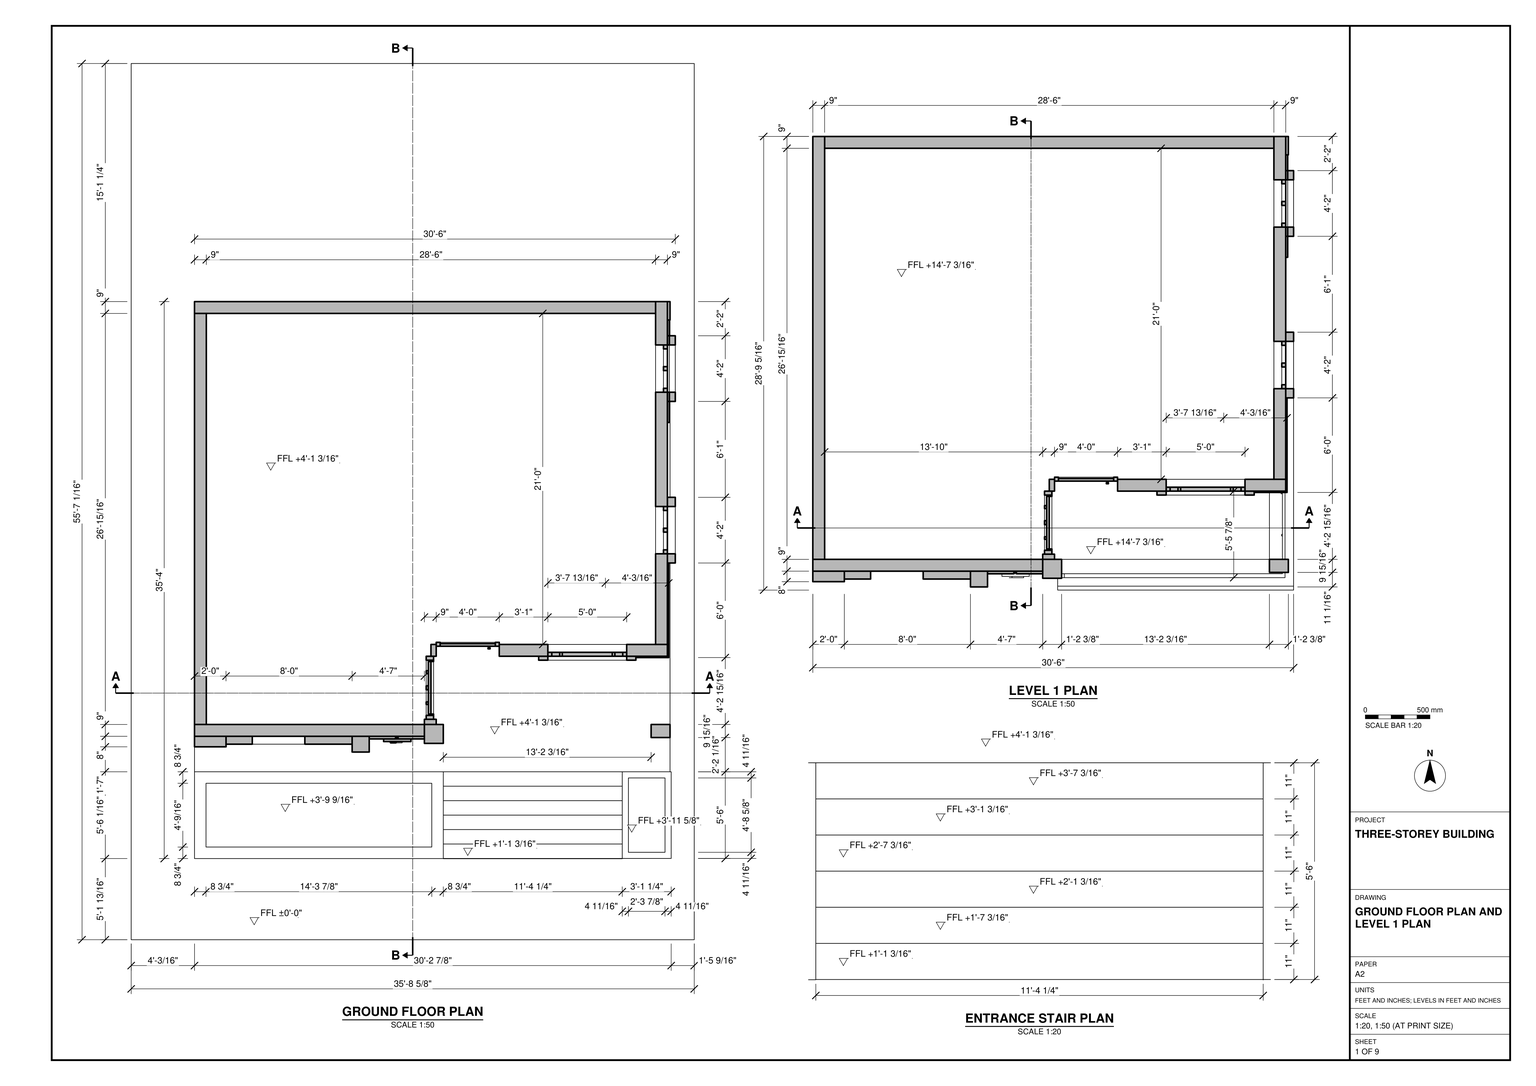
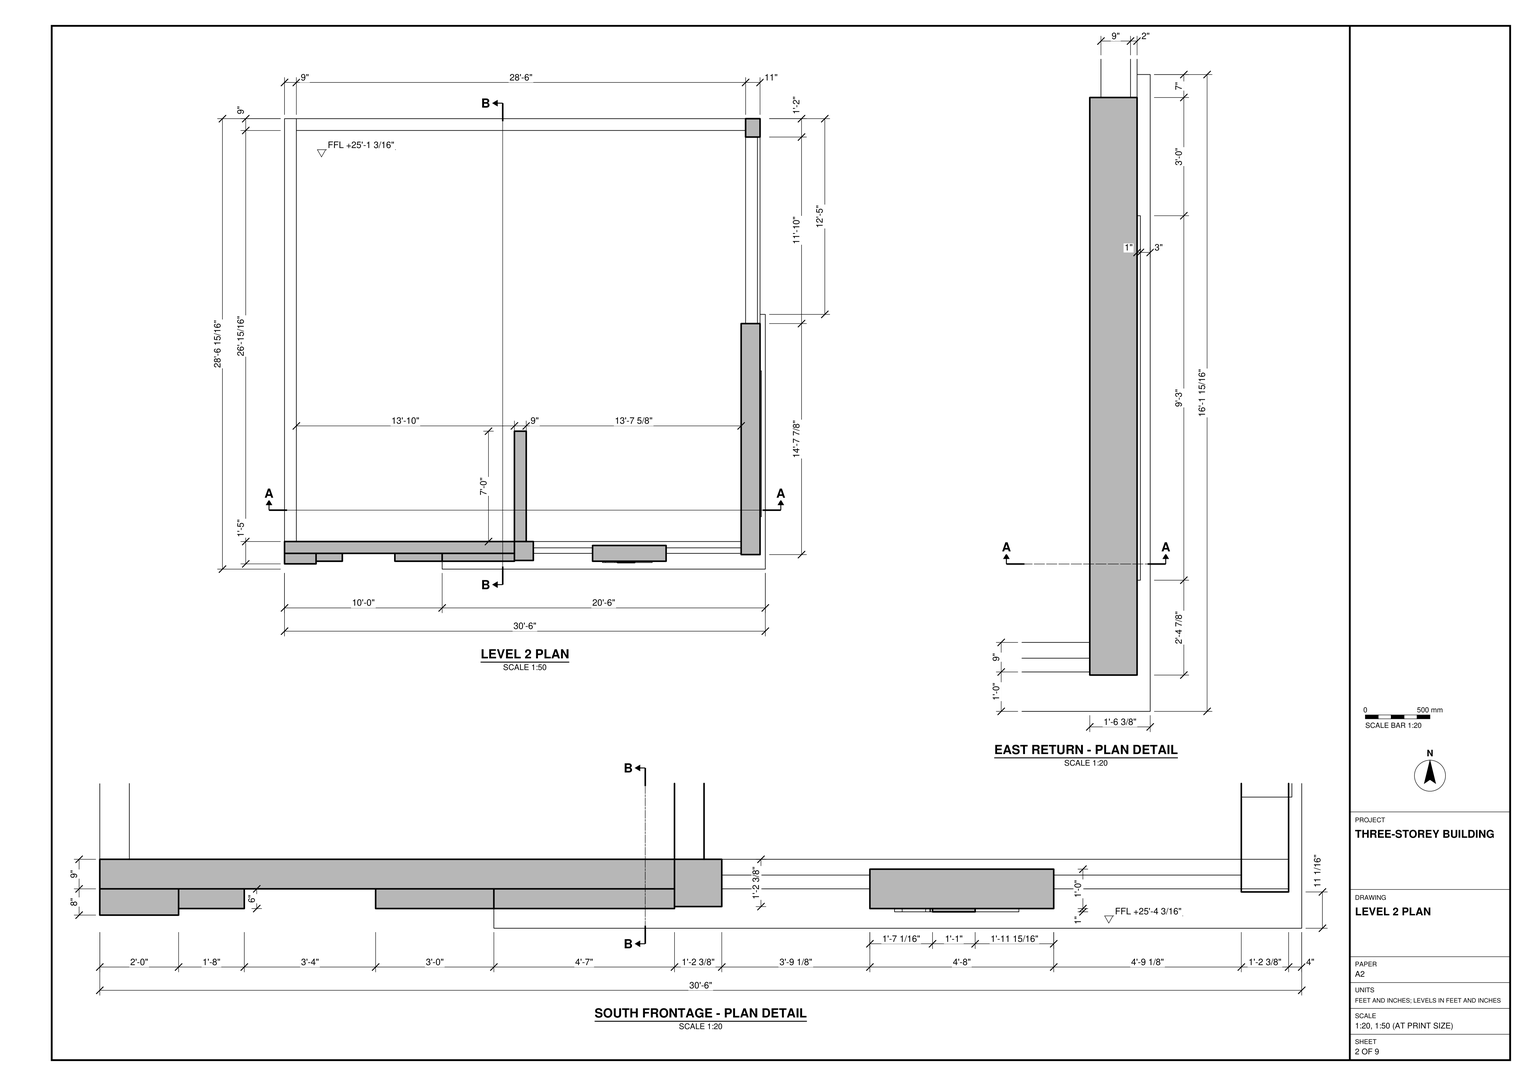
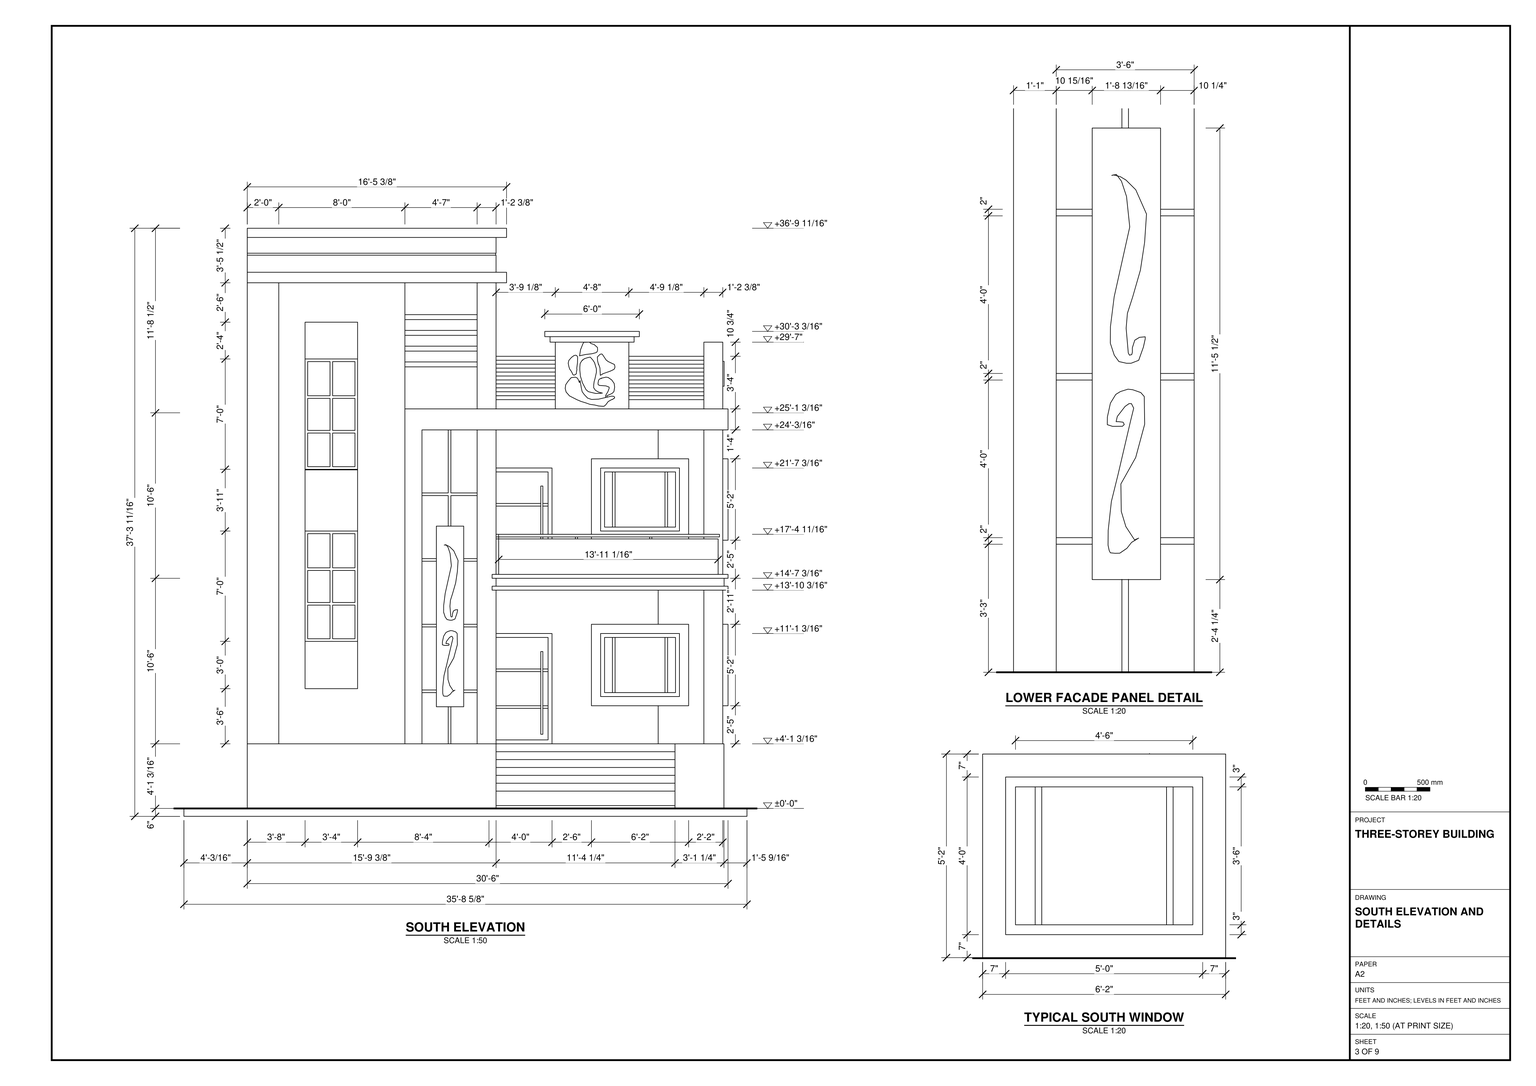
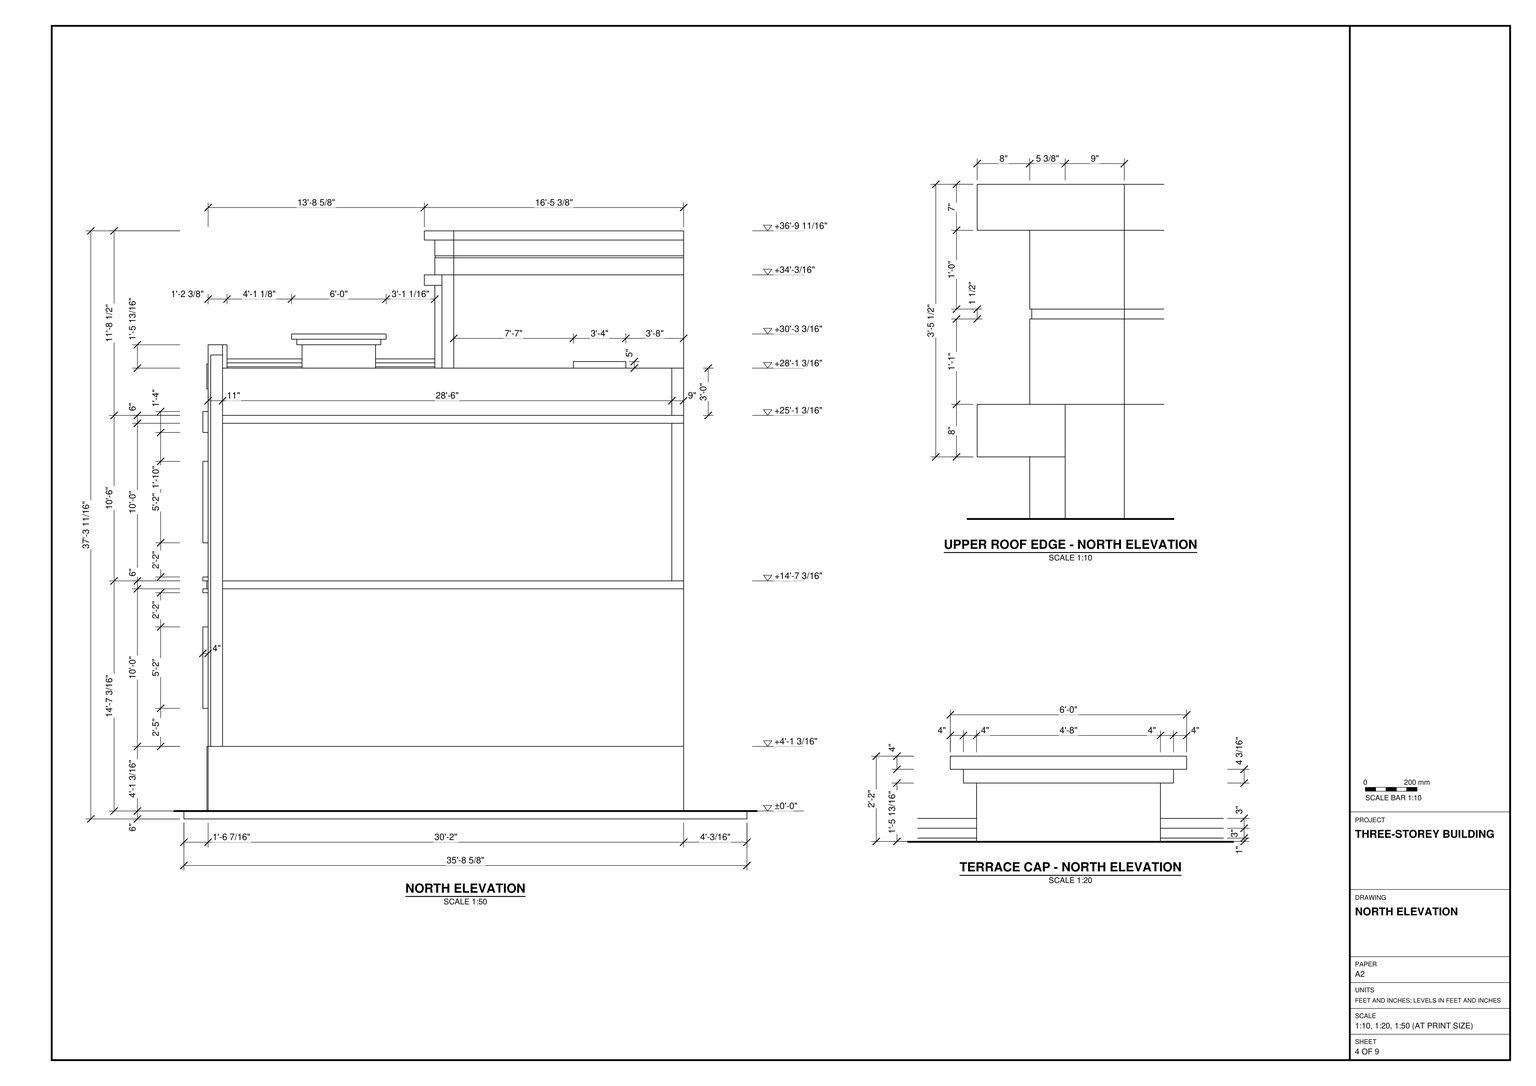
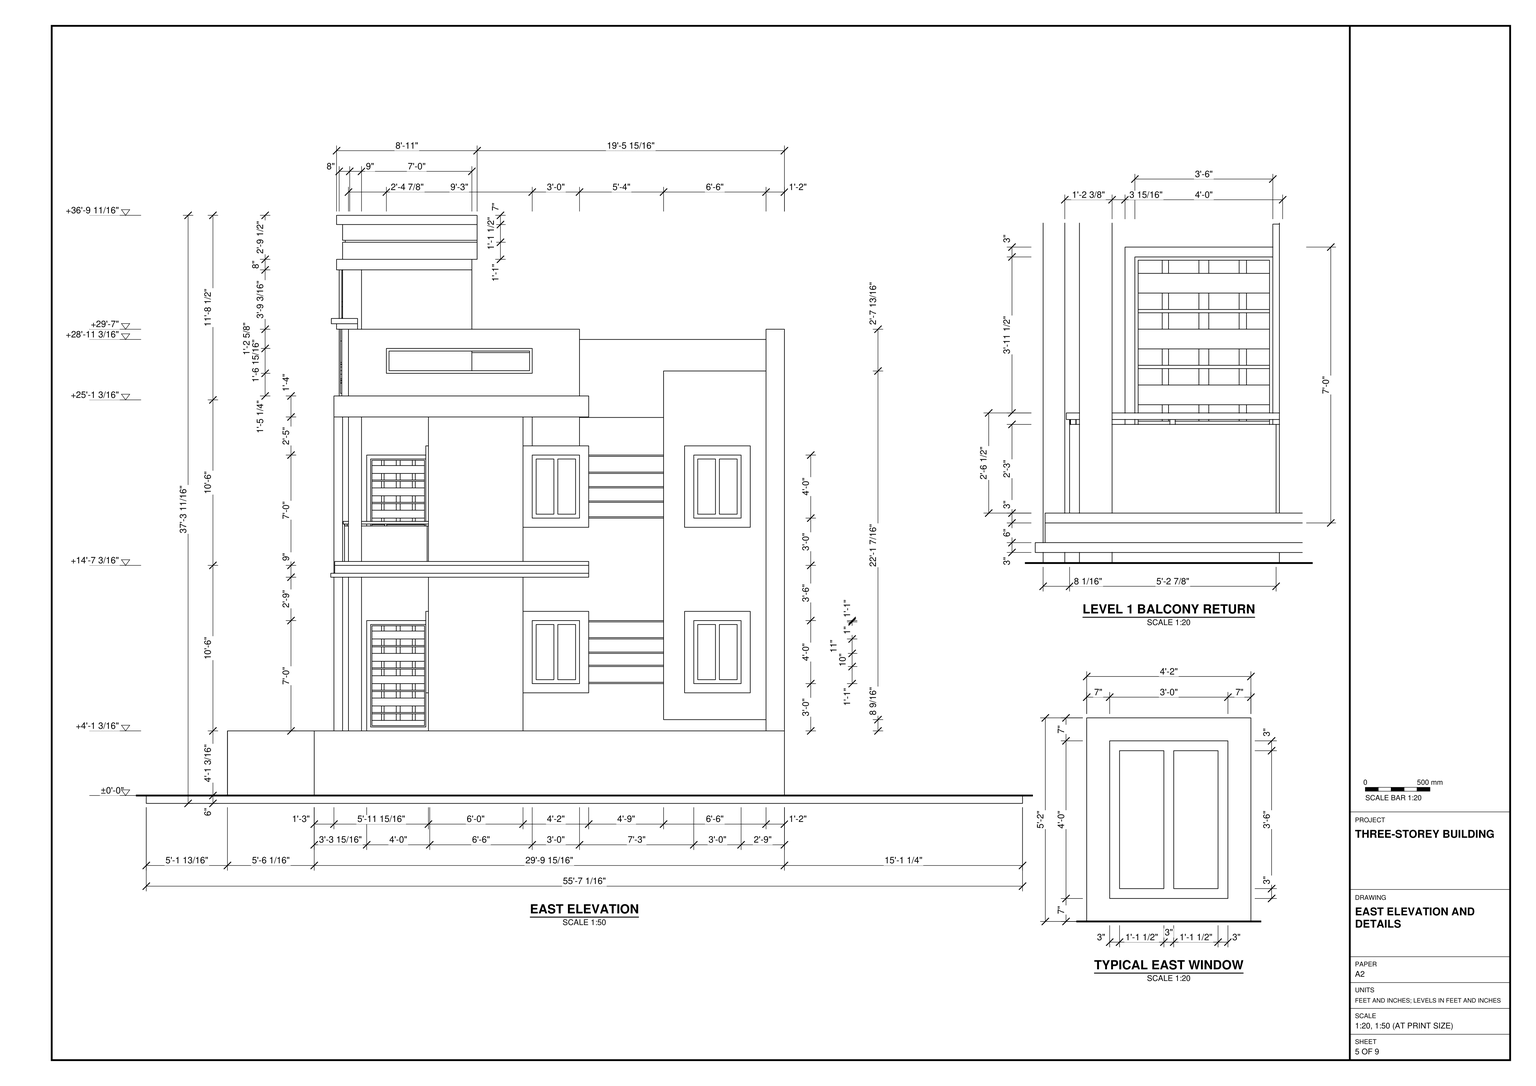
Build the three-storey building and its site base in SketchUp from task_files/diagram_01.pdf. Work in feet and inches. The overall model, including the base, is 35'-8 5/8" wide by 55'-7 1/16" deep by 37'-3 11/16" high. Use ±0'-0" as the ground datum, +14'-7 3/16" for Level 1 and +25'-1 3/16" for Level 2. The ground-floor entrance landing is raised to +4'-1 3/16" above the datum.

Lay out the walls and floor slabs from the plans, using the wall thicknesses shown, including the 9" perimeter walls where dimensioned. On the south side, model the broad entrance stair between its flanking raised sections. Set the entrance wall back from the tall left-hand bay and carry this recess through to the balcony above. Fit the doors and framed windows into the wall openings, including the stacked divided windows in the tall bay and the windows along the east wall. Model the balcony edge, the flat roof terrace, its horizontal rails and capped front panel, and the taller banded frontage and east return shown in the details.

Keep shell elements such as walls, slabs and roof separate as groups or components. Do the same for each furniture or joinery piece shown, and use components for repeated parts. Decor and loose items shown may be represented by any suitable library components. Save one SketchUp model as output_files/three_storey_building_with_raised_entrance.skp.

# SketchUp Ruby script. Lengths in inches.
U = 1.inch
M = Sketchup.active_model
def pt(a) = Geom::Point3d.new(a.map { |v| v * U })
def face(e, loops, mat)
  f = e.add_face(loops[0].map { |a| pt(a) })
  loops[1..].each { |l| e.add_face(l.map { |a| pt(a) }).erase! }
  f.material = f.back_material = mat if mat
  f
end
# faces: each face lists its corners as indices into pts; further lists are holes
def faces(e, pts, list, mat = nil) = list.each { |f| face(e, (f[0].is_a?(Array) ? f : [f]).map { |l| l.map { |i| pts[i] } }, mat) }
# xy, xz, yz: faces in a plane at the given z, y or x. An outline is a flat list of corners, or four numbers for a rectangle; further outlines are holes
def ring(l) = l.size == 4 ? [[l[0], l[1]], [l[2], l[1]], [l[2], l[3]], [l[0], l[3]]] : l.each_slice(2).to_a
def flat(e, list, mat, &to3) = list.each { |f| face(e, (f[0].is_a?(Array) ? f : [f]).map { |l| ring(l).map { |u, v| to3.(u, v) } }, mat) }
def xy(e, z, list, mat = nil) = flat(e, list, mat) { |x, y| [x, y, z] }
def xz(e, y, list, mat = nil) = flat(e, list, mat) { |x, z| [x, y, z] }
def yz(e, x, list, mat = nil) = flat(e, list, mat) { |y, z| [x, y, z] }
def lines(e, pts, list) = list.each { |a, b| e.add_line(pt(pts[a]), pt(pts[b])) }
# prism: a flat outline (further loops are holes) pulled along v
def prism(e, loops, v, mat = nil)
  f = face(e, loops, mat); d = Geom::Vector3d.new(v.map { |x| x * U })
  f.pushpull(f.normal.samedirection?(d) ? d.length : -d.length)
end
def box(e, o, s, mat = nil) = prism(e, [[o, [o[0] + s[0], o[1], o[2]], [o[0] + s[0], o[1] + s[1], o[2]], [o[0], o[1] + s[1], o[2]]]], [0, 0, s[2]], mat)
def at(x, y, z, deg = 0) = Geom::Transformation.translation(pt([x, y, z])) * Geom::Transformation.rotation(ORIGIN, Z_AXIS, deg.degrees)
def axes(o, x, y, z) = Geom::Transformation.new([*x, 0, *y, 0, *z, 0, *pt(o).to_a, 1])
def part(name) = M.definitions.add(name)
# library, detail: a bought-in or finely detailed component or shape, given as its bounding box
def library(name, o, s) = part(name).tap { |d| box(d.entities, o, s) }
def detail(e, o, s) = box(e.add_group.entities, o, s)
def put(e, d, t, mat = nil) = e.add_instance(d, t).tap { |i| i.material = mat if mat }
def group(e, t, mat = nil) = e.add_group.tap { |g| g.transformation = t; g.material = mat if mat }.entities
root = M.entities
M.materials.add("[Aluminum]").color = [179, 179, 179]
M.materials.add("[Color C08]").color = [102, 51, 0]
M.materials.add("[Color D05]").color = [255, 191, 0]
M.materials.add("[Color L16]").color = [102, 0, 51]
M.materials.add("[Color M00]").color = [255, 255, 255]
M.materials.add("[Color M09]").color = [0, 0, 0]
M.materials.add("[Field Rectangle Tile]").color = [196, 189, 179]
M.materials.add("[Grass Dark Green]").color = [106, 157, 55]
M.materials.add("[Metal Aluminum Anodized]").color = [202, 209, 219]
M.materials.add("[Translucent Glass Gray]").color = [255, 255, 255]
M.materials["[Translucent Glass Gray]"].alpha = 0.5
M.materials.add("[Translucent Glass Tinted]").color = [8, 201, 241]
M.materials["[Translucent Glass Tinted]"].alpha = 0.48
M.materials.add("[Wood Cherry Original]").color = [152, 86, 42]
c1 = part("Group\#13")
prism(c1.entities,[[[74,0,62],[0,0,62],[0,0,0],[74,0,0]],[[67,0,7],[7,0,7],[7,0,55],[67,0,55]]],[0,3,0])
c2 = part("Group\#14")
prism(c2.entities,[[[0,3,0],[0,3,84],[48,3,84],[48,3,0]],[[3,3,81],[3,3,3],[45,3,3],[45,3,81]]],[0,-3,0])
c3 = part("Group\#15")
prism(c3.entities,[[[42,2,0],[42,2,78],[42,0,78],[42,0,54],[42,1,54],[42,1,52],[42,0,52],[42,0,26],[42,1,26],[42,1,24],[42,0,24],[42,0,0]]],[-42,0,0])
c4 = part("Group\#16")
prism(c4.entities,[[[0,3,0],[0,3,48],[60,3,48],[60,3,0]],[[11,3,3],[49,3,3],[49,3,45],[11,3,45]],[[9,3,3],[9,3,45],[3,3,45],[3,3,3]],[[51,3,45],[51,3,3],[57,3,3],[57,3,45]]],[0,-3,0])
c5 = part("Group\#17")
prism(c5.entities,[[[54,0.23,0.01],[54,0.3125,0],[54,0.39,0.01],[54,0.47,0.04],[54,0.53,0.09],[54,0.58,0.16],[54,0.61,0.23],[54,0.625,0.3125],[54,0.61,0.39],[54,0.58,0.47],[54,0.53,0.53],[54,0.47,0.58],[54,0.39,0.61],[54,0.3125,0.625],[54,0.23,0.61],[54,0.16,0.58],[54,0.09,0.53],[54,0.04,0.47],[54,0.01,0.39],[54,0,0.3125],[54,0.01,0.23],[54,0.04,0.16],[54,0.09,0.09],[54,0.16,0.04]]],[-54,0,0])
c6 = part("Group\#18")
xz(c6.entities,0,[[0,0,54,42]])
c7 = part("Group\#19")
prism(c7.entities,[[[1.5625,2,61.21],[1.5625,2,63],[1.5625,0,63],[1.5625,0,0],[1.5625,2,0],[1.5625,2,1.79],[1.5625,0.79,1.79],[1.5625,0.79,61.21]]],[-1.5625,0,0])
c8 = part("Group\#20")
prism(c8.entities,[[[0,75.9375,120],[0,75.9375,84],[0,27.9375,84],[0,27.9375,0],[0,24,0],[0,24,120]]],[9,0,0])
c9 = part("Group\#21")
prism(c9.entities,[[[-2.625,0,84],[-2.625,48,84],[-2.625,48,0],[-2.625,0,0]],[[-2.625,45,3],[-2.625,45,81],[-2.625,3,81],[-2.625,3,3]]],[5.625,0,0])
c10 = part("Group\#22")
xy(c10.entities,0,[[0,0,2,42]])
xy(c10.entities,1,[[0,1,2,41],[-3.625,19.5,0,22.5]])
xy(c10.entities,77,[[0,1,2,19.5],[-3.625,19.5,0,22.5],[0,19.5,2,22.5],[0,22.5,2,41]])
xy(c10.entities,78,[[0,0,2,42]])
xz(c10.entities,0,[[0,0,2,78]])
xz(c10.entities,1,[[0,1,2,77]])
xz(c10.entities,41,[[0,1,2,77]])
xz(c10.entities,42,[[0,0,2,78]])
yz(c10.entities,0,[[[0,0,42,78],[1,1,41,77]]])
yz(c10.entities,2,[[[0,0,42,78],[1,1,41,77]]])
c11 = library("Group\#23",[-1.625,1,1],[3.625,40,80.9375])
c12 = part("Group\#48")
prism(c12.entities,[[[0.6,1.6,0],[0.8125,1.625,0],[1.02,1.6,0],[1.22,1.52,0],[1.39,1.39,0],[1.52,1.22,0],[1.6,1.02,0],[1.625,0.8125,0],[1.6,0.6,0],[1.52,0.41,0],[1.39,0.24,0],[1.22,0.11,0],[1.02,0.03,0],[0.8125,0,0],[0.6,0.03,0],[0.41,0.11,0],[0.24,0.24,0],[0.11,0.41,0],[0.03,0.6,0],[0,0.8125,0],[0.03,1.02,0],[0.11,1.22,0],[0.24,1.39,0],[0.41,1.52,0]]],[0,0,28.5])
c13 = part("Group\#64")
box(c13.entities,[0,0,2.1875],[55,6,3.76])
c14 = part("Group\#58")
prism(c14.entities,[[[40,3,84],[40,3,0],[0,3,0],[0,3,84]],[[19,3,56],[19,3,82],[2,3,82],[2,3,56]],[[38,3,82],[21,3,82],[21,3,56],[38,3,56]],[[19,3,27.6],[2,3,27.6],[2,3,2],[19,3,2]],[[38,3,2],[38,3,27.6],[21,3,27.6],[21,3,2]],[[19,3,29.6],[19,3,54],[2,3,54],[2,3,29.6]],[[38,3,29.6],[38,3,54],[21,3,54],[21,3,29.6]]],[0,-3,0])
c15 = part("Group\#78")
box(c15.entities,[0,0,0],[158.2,4.1875,3])
c16 = library("Group\#92",[0,0,0],[37.85,2,48.8125])
prism(root,[[[202.41,150.87,93.57],[205.07,150.87,89.51],[206.32,150.87,90.07],[204.17,150.87,88.78],[202.73,150.87,86.95],[200.5625,150.87,85.47],[199.13,150.87,85.44],[197.69,150.87,85.59],[197.34,150.87,86.3],[196.99,150.87,87.91],[197.03,150.87,92.39],[198,150.87,101.17],[200.03,150.87,109.4],[203.89,150.87,125.92],[204.8,150.87,129.63],[204.1,150.87,131.03],[203.4,150.87,131.02],[202.15,150.87,130.13],[199.8125,150.87,127.11],[199.44,150.87,125.52],[200.16,150.87,125.53],[201.58,150.87,125.37],[201.93,150.87,124.66],[201.39,150.87,124.13],[200.68,150.87,124.12],[198.36,150.87,124.1],[196.76,150.87,124.61],[196.77,150.87,125.32],[196.78,150.87,126.91],[197.71,150.87,131.15],[199.33,150.87,133.81],[200.76,150.87,134.7],[203.07,150.87,135.42],[204.49,150.87,135.25],[206.96,150.87,134.39],[208.02,150.87,133.17],[208.14,150.87,124.73],[205.41,150.87,114.62],[200.9,150.87,106.57],[201.02,150.87,98.19]]],[0,-1,0],"[Aluminum]")
xz(root,149.87,[[202.6,143.3125,204.01,143.32,206.32,144.21,207.76,148.23,208.3,150.68,208.3,151.375,206.54,151.2,205.12,150.32,204.4,148.05,204.39,146.65,204.21,145.95,203.5,145.77,203.15,146.47,202.5,153.98,202.88,158.51,204.51,163.55,206.85,171.69,208.13,180.14,208.71,188.74,205.43,196.14,202.48,199.08,200.73,200.13,199.87,200.35,201.07,198.76,202.61,194.11,203.6,184.82,198.86,163.56,197.72,154.49,197.68,149.42,198.89,145.75,200.3,143.83]],"[Aluminum]")
xz(root,150.87,[[202.6,143.3125,200.3,143.83,198.89,145.75,197.68,149.42,197.72,154.49,198.86,163.56,203.6,184.82,202.61,194.11,201.07,198.76,199.87,200.35,200.73,200.13,202.48,199.08,205.43,196.14,208.71,188.74,208.13,180.14,206.85,171.69,204.51,163.55,202.88,158.51,202.5,153.98,203.15,146.47,203.5,145.77,204.21,145.95,204.39,146.65,204.4,148.05,205.12,150.32,206.54,151.2,208.3,151.375,208.3,150.68,207.76,148.23,206.32,144.21,204.01,143.32],[199.87,200.35,198.72,200.65,199.51,200.83],[198.1,200.51,198.63,200.67,198.72,200.65]])
yz(root,208.3,[[149.87,150.68,150.87,151.375]])
p = [[200.3,150.87,143.83],[202.6,150.87,143.3125],[202.6,149.87,143.3125],[200.3,149.87,143.83],[204.01,150.87,143.32],[204.01,149.87,143.32],
  [206.32,150.87,144.21],[206.32,149.87,144.21],[198.89,150.87,145.75],[198.89,149.87,145.75],[207.76,150.87,148.23],[207.76,149.87,148.23],
  [197.68,150.87,149.42],[197.68,149.87,149.42],[203.5,150.87,145.77],[203.15,150.87,146.47],[203.15,149.87,146.47],[203.5,149.87,145.77],
  [204.21,150.87,145.95],[204.21,149.87,145.95],[204.39,150.87,146.65],[204.39,149.87,146.65],[202.5,150.87,153.98],[202.5,149.87,153.98],
  [204.4,150.87,148.05],[204.4,149.87,148.05],[205.12,150.87,150.32],[205.12,149.87,150.32],[208.3,150.87,150.68],[208.3,149.87,150.68],
  [197.72,150.87,154.49],[197.72,149.87,154.49],[206.54,150.87,151.2],[206.54,149.87,151.2],[208.3,150.87,151.375],[208.3,149.87,151.375],
  [202.88,150.87,158.51],[202.88,149.87,158.51],[198.86,150.87,163.56],[198.86,149.87,163.56],[204.51,150.87,163.55],[204.51,149.87,163.55],
  [203.6,150.87,184.82],[203.6,149.87,184.82],[206.85,150.87,171.69],[206.85,149.87,171.69],[208.13,150.87,180.14],[208.13,149.87,180.14],
  [208.71,150.87,188.74],[208.71,149.87,188.74],[202.61,150.87,194.11],[202.61,149.87,194.11],[205.43,150.87,196.14],[205.43,149.87,196.14],
  [201.07,150.87,198.76],[201.07,149.87,198.76],[202.48,150.87,199.08],[202.48,149.87,199.08],[199.87,150.87,200.35],[199.87,149.87,200.35],
  [200.73,150.87,200.13],[200.73,149.87,200.13]]
faces(root,p,[[0,1,2,3],[1,4,5,2],[4,6,7,5],[8,0,3,9],[6,10,11,7],[12,8,9,13],[14,15,16,17],[18,14,17,19],
  [20,18,19,21],[15,22,23,16],[24,20,21,25],[26,24,25,27],[10,28,29,11],[30,12,13,31],[32,26,27,33],[34,32,33,35],
  [22,36,37,23],[38,30,31,39],[36,40,41,37],[42,38,39,43],[40,44,45,41],[44,46,47,45],[46,48,49,47],[50,42,43,51],
  [48,52,53,49],[54,50,51,55],[52,56,57,53],[58,54,55,59],[56,60,61,57],[60,58,59,61]])
g1 = group(root,at(48.21,125.8,37.2))
box(g1,[0,2.0625,-37.2],[362,357.9375,49.2])
g2 = group(root,at(399.21,125.8,49.2))
xy(g2,0,[[0,99,9,360]])
xy(g2,36,[[0,168,9,204],[8,211,9,268],[0,291,9,327]])
xy(g2,37,[[8,211,9,268]])
xy(g2,49,[[8,211,9,268]])
xy(g2,50,[[8,211,9,268]])
xy(g2,59,[[8,211,9,268]])
xy(g2,60,[[8,211,9,268]])
xy(g2,70,[[8,211,9,268]])
xy(g2,71,[[8,211,9,268]])
xy(g2,83,[[8,211,9,268]])
xy(g2,84,[[0,168,9,204],[8,211,9,268],[0,291,9,327]])
xy(g2,162,[[0,168,9,204],[8,211,9,268],[0,291,9,327]])
xy(g2,163,[[8,211,9,268]])
xy(g2,174,[[8,211,9,268]])
xy(g2,175,[[8,211,9,268]])
xy(g2,185,[[8,211,9,268]])
xy(g2,186,[[8,211,9,268]])
xy(g2,196,[[8,211,9,268]])
xy(g2,197,[[8,211,9,268]])
xy(g2,209,[[8,211,9,268]])
xy(g2,210,[[0,168,9,204],[8,211,9,268],[0,291,9,327]])
xy(g2,269.23,[[0,99,9,170.625]])
xy(g2,298,[[0,170.625,9,360]])
xz(g2,99,[[0,0,9,269.23]])
xz(g2,168,[[0,36,9,84],[0,162,9,210]])
xz(g2,170.625,[[0,269.23,9,298]])
xz(g2,204,[[0,36,9,84],[0,162,9,210]])
xz(g2,211,[[8,36,9,37],[8,49,9,50],[8,59,9,60],[8,70,9,71],[8,83,9,84],
  [8,162,9,163],[8,174,9,175],[8,185,9,186],[8,196,9,197],[8,209,9,210]])
xz(g2,268,[[8,36,9,37],[8,49,9,50],[8,59,9,60],[8,70,9,71],[8,83,9,84],
  [8,162,9,163],[8,174,9,175],[8,185,9,186],[8,196,9,197],[8,209,9,210]])
xz(g2,291,[[0,36,9,84],[0,162,9,210]])
xz(g2,327,[[0,36,9,84],[0,162,9,210]])
xz(g2,360,[[0,0,9,298]])
yz(g2,0,[[[99,0,99,269.23,170.625,269.23,170.625,298,360,298,360,0],[291,36,327,84],[168,36,204,84],[291,162,327,210],[168,162,204,210]]])
yz(g2,8,[[211,36,268,37],[211,49,268,50],[211,59,268,60],[211,70,268,71],[211,83,268,84],
  [211,162,268,163],[211,174,268,175],[211,185,268,186],[211,196,268,197],[211,209,268,210]])
yz(g2,9,[[[99,0,360,0,360,298,170.625,298,170.625,269.23,99,269.23],[291,36,327,84],[168,36,204,84],[168,162,204,210],[291,162,327,210],[211,209,268,210],[211,196,268,197],[211,185,268,186],[211,174,268,175],[211,162,268,163],[211,83,268,84],[211,70,268,71],[211,59,268,60],[211,49,268,50],[211,36,268,37]]])
p = [[9,161,117],[9,161,0]]
lines(g2,p,[[0,1]])
g3 = group(root,at(408.21,286.8,78.2))
prism(g3,[[[0,0,0],[0,0,62],[0,50,62],[0,50,0]],[[0,43,55],[0,7,55],[0,7,7],[0,43,7]]],[6,0,0])
g4 = group(root,at(408.21,409.8,78.2))
prism(g4,[[[0,0,0],[0,0,62],[0,50,62],[0,50,0]],[[0,43,55],[0,7,55],[0,7,7],[0,43,7]]],[6,0,0])
g5 = group(root,at(405.21,416.8,85.2),"[Color M09]")
prism(g5,[[[0,0,0],[0,0,48],[0,36,48],[0,36,0]],[[0,19.5,45],[0,19.5,3],[0,33,3],[0,33,45]],[[0,16.5,45],[0,3,45],[0,3,3],[0,16.5,3]]],[3,0,0])
g6 = group(root,at(408.21,436.3,88.2),"[Translucent Glass Gray]")
yz(g6,0,[[0,0,13.5,42]])
g7 = group(root,at(408.21,419.8,88.2),"[Translucent Glass Gray]")
yz(g7,0,[[0,0,13.5,42]])
g8 = group(root,at(405.21,293.8,85.2),"[Color M09]")
prism(g8,[[[0,36,48],[0,36,0],[0,0,0],[0,0,48]],[[0,19.5,45],[0,19.5,3],[0,33,3],[0,33,45]],[[0,16.5,45],[0,3,45],[0,3,3],[0,16.5,3]]],[3,0,0])
g9 = group(root,at(408.21,313.3,88.2),"[Translucent Glass Gray]")
yz(g9,0,[[0,0,13.5,42]])
g10 = group(root,at(408.21,296.8,88.2),"[Translucent Glass Gray]")
yz(g10,0,[[0,0,13.5,42]])
g11 = group(root,at(228.21,215.8,49.2))
prism(g11,[[[4,9,0],[0,9,0],[0,9,120],[180,9,120],[180,9,0],[52,9,0],[52,9,84],[4,9,84]],[[149,9,84],[89,9,84],[89,9,36],[149,9,36]]],[0,-9,0])
put(root,c1,at(310.21,212.8,78.2))
put(root,c2,at(232.21,223.43,49.2),"[Wood Cherry Original]")
put(root,c3,at(235.21,223.43,52.2),"[Wood Cherry Original]")
put(root,c4,at(317.21,215.8,85.2),"[Color M09]")
put(root,c5,at(320.21,216.99,127.07),"[Color M09]")
put(root,c5,at(320.21,216.99,124.07),"[Color M09]")
put(root,c5,at(320.21,216.99,121.07),"[Color M09]")
put(root,c5,at(320.21,216.99,118.07),"[Color M09]")
put(root,c5,at(320.21,216.99,115.07),"[Color M09]")
put(root,c5,at(320.21,216.99,112.07),"[Color M09]")
put(root,c5,at(320.21,216.99,109.07),"[Color M09]")
put(root,c5,at(320.21,216.99,106.07),"[Color M09]")
put(root,c5,at(320.21,216.99,103.07),"[Color M09]")
put(root,c5,at(320.21,216.99,100.07),"[Color M09]")
put(root,c5,at(320.21,216.99,97.07),"[Color M09]")
put(root,c5,at(320.21,216.99,94.07),"[Color M09]")
put(root,c5,at(320.21,216.99,91.07),"[Color M09]")
put(root,c6,at(320.21,218.8,88.2))
put(root,c7,at(271.67,221.43,56.47),"[Metal Aluminum Anodized]")
put(root,c8,at(223.21,139.87,49.2))
put(root,c9,at(227.21,167.8,49.2))
put(root,c10,at(228.21,170.8,52.2))
put(root,c11,at(226.21,170.8,52.2))
g12 = group(root,at(48.21,154.87,49.2))
prism(g12,[[[0,0,0],[175,0,0],[175,0,359],[0,0,359]],[[44,0,293],[84,0,293],[84,0,208.5625],[44,0,208.5625]],[[84,0,78],[44,0,78],[44,0,162],[84,0,162]]],[0,9,0])
g13 = group(root,at(48.21,476.8,49.2))
box(g13,[0,0,0],[351,9,120])
g14 = group(root,at(48.21,163.87,49.2))
box(g14,[0,0,0],[9,312.9375,120])
g15 = group(root,at(48.21,163.87,169.2))
prism(g15,[[[0,0,0],[0,321.9375,0],[351,321.9375,0],[351,60.9375,0],[360,60.9375,0],[360,172.9375,0],[363,172.9375,0],[363,-20.4,0],[189.4,-20.4,0],[189.4,0,0]]],[0,0,6],"[Wood Cherry Original]")
put(root,c9,at(227.21,167.8,175.2))
put(root,c5,at(320.21,216.99,232.07),"[Color M09]")
put(root,c1,at(310.21,212.8,204.2))
g16 = group(root,at(228.21,215.8,175.2))
prism(g16,[[[4,9,0],[0,9,0],[0,9,120],[180,9,120],[180,9,0],[52,9,0],[52,9,84],[4,9,84]],[[149,9,84],[89,9,84],[89,9,36],[149,9,36]]],[0,-9,0])
put(root,c4,at(317.21,215.8,211.2),"[Color M09]")
put(root,c2,at(232.21,223.43,175.2),"[Wood Cherry Original]")
put(root,c5,at(320.21,216.99,247.07),"[Color M09]")
put(root,c5,at(320.21,216.99,217.07),"[Color M09]")
put(root,c10,at(228.21,170.8,178.2))
put(root,c5,at(320.21,216.99,253.07),"[Color M09]")
put(root,c3,at(235.21,223.43,178.2),"[Wood Cherry Original]")
put(root,c6,at(320.21,218.8,214.2))
put(root,c5,at(320.21,216.99,220.07),"[Color M09]")
put(root,c7,at(271.67,221.43,182.47),"[Metal Aluminum Anodized]")
put(root,c5,at(320.21,216.99,241.07),"[Color M09]")
put(root,c5,at(320.21,216.99,229.07),"[Color M09]")
put(root,c5,at(320.21,216.99,226.07),"[Color M09]")
put(root,c5,at(320.21,216.99,244.07),"[Color M09]")
put(root,c5,at(320.21,216.99,238.07),"[Color M09]")
put(root,c11,at(226.21,170.8,178.2))
put(root,c5,at(320.21,216.99,235.07),"[Color M09]")
put(root,c5,at(320.21,216.99,250.07),"[Color M09]")
put(root,c8,at(223.21,139.87,175.2))
put(root,c5,at(320.21,216.99,223.07),"[Color M09]")
g17 = group(root,at(408.21,286.8,204.2))
prism(g17,[[[0,0,0],[0,0,62],[0,50,62],[0,50,0]],[[0,7,55],[0,7,7],[0,43,7],[0,43,55]]],[6,0,0])
g18 = group(root,at(408.21,409.8,204.2))
prism(g18,[[[0,0,62],[0,50,62],[0,50,0],[0,0,0]],[[0,43,55],[0,7,55],[0,7,7],[0,43,7]]],[6,0,0])
g19 = group(root,at(405.21,293.8,211.2),"[Color M09]")
prism(g19,[[[3,0,0],[3,36,0],[3,36,48],[3,0,48]],[[3,19.5,3],[3,19.5,45],[3,33,45],[3,33,3]],[[3,3,45],[3,16.5,45],[3,16.5,3],[3,3,3]]],[-3,0,0])
g20 = group(root,at(408.21,313.3,214.2),"[Translucent Glass Gray]")
yz(g20,0,[[0,0,13.5,42]])
g21 = group(root,at(408.21,296.8,214.2),"[Translucent Glass Gray]")
yz(g21,0,[[0,0,13.5,42]])
g22 = group(root,at(405.21,416.8,211.2),"[Color M09]")
prism(g22,[[[0,36,48],[0,36,0],[0,0,0],[0,0,48]],[[0,19.5,45],[0,19.5,3],[0,33,3],[0,33,45]],[[0,16.5,45],[0,3,45],[0,3,3],[0,16.5,3]]],[3,0,0])
g23 = group(root,at(408.21,436.3,214.2),"[Translucent Glass Gray]")
yz(g23,0,[[0,0,13.5,42]])
g24 = group(root,at(408.21,419.8,214.2),"[Translucent Glass Gray]")
yz(g24,0,[[0,0,13.5,42]])
g25 = group(root,at(48.21,163.87,175.2))
box(g25,[0,0,0],[9,321.9375,120])
g26 = group(root,at(57.21,476.8,175.2))
box(g26,[0,0,0],[342,9,120])
g27 = group(root,at(48.21,163.87,295.2))
prism(g27,[[[189.4,0,0],[0,0,0],[0,321.9375,0],[351,321.9375,0],[351,60.9375,0],[362,60.9375,0],[362,-9,0],[189.4,-9,0]]],[0,0,6])
g28 = group(root,at(232.21,140.47,166.2))
prism(g28,[[[0,75.34,0],[176,75.34,0],[176,196.34,0],[182,196.34,0],[182,0,0],[2.4,0,0],[2.4,10.0625,0],[0,10.0625,0]]],[0,0,3])
g29 = group(root,at(223.21,149.47,49.2),"[Color D05]")
box(g29,[0,0,0],[14.4,14.4,359])
g30 = group(root,at(237.61,143.47,175.2))
xy(g30,0,[[-3,0,-3,6,0,6,0,20.4,167.6,20.4,167.6,9,176.6,9,176.6,0],[167.6,9,167.6,20.4,158.2,20.4,158.2,72.34,170.6,72.34,170.6,193.34,176.6,193.34,176.6,9]])
xy(g30,3,[[-3,0,176.6,0,176.6,193.34,170.6,193.34,170.6,72.34,158.2,72.34,158.2,20.4,0,20.4,0,6,-3,6]])
xz(g30,0,[[-3,0,176.6,3]])
xz(g30,6,[[-3,0,0,3]])
xz(g30,20.4,[[0,0,158.2,3]])
xz(g30,72.34,[[158.2,0,170.6,3]])
xz(g30,193.34,[[170.6,0,176.6,3]])
yz(g30,-3,[[0,0,6,3]])
yz(g30,0,[[6,0,20.4,3]])
yz(g30,158.2,[[20.4,0,72.34,3]])
yz(g30,170.6,[[72.34,0,193.34,3]])
yz(g30,176.6,[[0,0,193.34,3]])
g31 = group(root,at(237.61,150.92,178.2))
box(g31,[0,0,0],[2,2,27])
g32 = group(root,at(395.8125,149.47,49.2),"[Color L16]")
xy(g32,0,[[0,4.46,14.4,14.4]])
xy(g32,217,[[12.4,144.34,14.4,180.34]])
xy(g32,252,[[0,14.4,0,180.34,12.4,180.34,12.4,144.34,14.4,144.34,14.4,14.4]])
xy(g32,272.23,[[0,33.34,14.4,144.34]])
xy(g32,291.18,[[0,33.34,14.4,144.34]])
xy(g32,305.79,[[0,4.46,14.4,180.34]])
xz(g32,4.46,[[0,0,14.4,305.79]])
xz(g32,14.4,[[0,0,14.4,252]])
xz(g32,33.34,[[0,272.23,14.4,291.18]])
xz(g32,144.34,[[12.4,217,14.4,252],[0,272.23,14.4,291.18]])
xz(g32,180.34,[[12.4,217,12.4,252,0,252,0,305.79,14.4,305.79,14.4,217]])
yz(g32,0,[[[4.46,0,4.46,305.79,180.34,305.79,180.34,252,14.4,252,14.4,0],[33.34,272.23,144.34,291.18]]])
yz(g32,12.4,[[144.34,217,180.34,252]])
yz(g32,14.4,[[[4.46,0,14.4,0,14.4,252,144.34,252,144.34,217,180.34,217,180.34,305.79,4.46,305.79],[33.34,272.23,144.34,291.18]]])
g33 = group(root,at(239.61,150.92,178.2),"[Translucent Glass Gray]")
xz(g33,0,[[0,0,167.0625,27]])
g34 = group(root,at(404.68,213.8,178.2))
box(g34,[0,0,0],[2,2,27])
g35 = group(root,at(406.68,150.92,178.2),"[Translucent Glass Gray]")
yz(g35,0,[[0,0,62.88,27]])
g36 = group(root,at(237.61,149.92,205.2),"[Metal Aluminum Anodized]")
xy(g36,0,[[0,1,2,3]])
xy(g36,1.5,[[0,0,2,1],[2,0,2,3,168.0625,3,168.0625,65.88,170.0625,65.88,170.0625,0],[0,1,2,3]])
xy(g36,3.5,[[0,0,2,3],[2,0,170.0625,0,170.0625,65.88,168.0625,65.88,168.0625,3,2,3]])
xz(g36,0,[[0,1.5,2,3.5],[2,1.5,170.0625,3.5]])
xz(g36,1,[[0,0,2,1.5]])
xz(g36,3,[[0,0,2,1.5],[0,1.5,2,3.5],[2,1.5,168.0625,3.5]])
xz(g36,65.88,[[168.0625,1.5,170.0625,3.5]])
yz(g36,0,[[1,0,3,1.5],[0,1.5,3,3.5]])
yz(g36,2,[[1,0,3,1.5],[0,1.5,3,3.5]])
yz(g36,168.0625,[[3,1.5,65.88,3.5]])
yz(g36,170.0625,[[0,1.5,65.88,3.5]])
put(root,c12,at(298.01,151.11,178.2))
put(root,c12,at(354.59,151.21,178.2))
put(root,c12,at(404.99,181.47,178.2))
g37 = group(root,at(168.21,142.87,49.2))
xy(g37,0,[[0,0,13,12]])
xy(g37,239,[[13,0,13,12,242,12,242,193.9375,246,193.9375,246,0]])
xy(g37,255,[[0,0,246,0,246,193.9375,242,193.9375,242,12,0,12]])
xz(g37,0,[[0,0,13,0,13,239,246,239,246,255,0,255]])
xz(g37,12,[[0,0,0,255,242,255,242,239,13,239,13,0]])
xz(g37,193.9375,[[242,239,246,255]])
yz(g37,0,[[0,0,12,255]])
yz(g37,13,[[0,0,12,239]])
yz(g37,242,[[12,239,193.9375,255]])
yz(g37,246,[[0,239,193.9375,255]])
g38 = group(root,at(181.21,153.87,49.2),"[Color C08]")
xy(g38,0,[[0,-1,0,1,42,1,42,-1,22,-1,22,0,20,0,20,-1]])
xy(g38,39,[[0,-1,20,0],[22,-1,42,0]])
xy(g38,41,[[0,-1,20,0],[22,-1,42,0]])
xy(g38,89,[[0,-1,20,0],[22,-1,42,0]])
xy(g38,91,[[0,-1,20,0],[22,-1,42,0]])
xy(g38,139,[[0,-1,20,0],[22,-1,42,0]])
xy(g38,141,[[0,-1,20,0],[22,-1,42,0]])
xy(g38,189,[[0,-1,20,0],[22,-1,42,0]])
xy(g38,191,[[0,-1,20,0],[22,-1,42,0]])
xy(g38,239,[[0,-1,20,-1,20,0,22,0,22,-1,42,-1,42,1,0,1]])
xz(g38,-1,[[0,0,20,39],[22,0,42,39],[0,41,20,89],[22,41,42,89],[0,91,20,139],
  [22,91,42,139],[0,141,20,189],[22,141,42,189],[0,191,20,239],[22,191,42,239]])
xz(g38,0,[[20,0,22,0,22,39,42,39,42,41,22,41,22,89,42,89,42,91,22,91,22,139,42,139,42,141,22,141,22,189,42,189,42,191,22,191,22,239,20,239,20,191,0,191,0,189,20,189,20,141,0,141,0,139,20,139,20,91,0,91,0,89,20,89,20,41,0,41,0,39,20,39]])
xz(g38,1,[[0,0,42,239]])
yz(g38,0,[[-1,0,-1,39,0,39,0,41,-1,41,-1,89,0,89,0,91,-1,91,-1,139,0,139,0,141,-1,141,-1,189,0,189,0,191,-1,191,-1,239,1,239,1,0]])
yz(g38,20,[[-1,0,0,39],[-1,41,0,89],[-1,91,0,139],[-1,141,0,189],[-1,191,0,239]])
yz(g38,22,[[-1,0,0,39],[-1,41,0,89],[-1,91,0,139],[-1,141,0,189],[-1,191,0,239]])
yz(g38,42,[[-1,0,1,0,1,239,-1,239,-1,191,0,191,0,189,-1,189,-1,141,0,141,0,139,-1,139,-1,91,0,91,0,89,-1,89,-1,41,0,41,0,39,-1,39]])
g39 = group(root,at(395.8125,182.8,321.43))
prism(g39,[[[0,0,0],[0,0,18.96],[0,111,18.96],[0,111,0]],[[0,2,16.96],[0,2,2],[0,109,2],[0,109,16.96]]],[15.4,0,0])
g40 = group(root,at(399.21,471.8,49.2))
prism(g40,[[[9,14,0],[9,14,298],[0,14,298],[0,14,305.79],[11,14,305.79],[11,14,0]]],[0,-14,0])
g41 = group(root,at(408.21,329.8,287.82),"[Color C08]")
xy(g41,0,[[0,0,2,64]])
xy(g41,35.375,[[0,64,2,142]])
xy(g41,59.375,[[0,0,2,142]])
xz(g41,0,[[0,0,2,35.375],[0,35.375,2,59.375]])
xz(g41,64,[[0,0,2,35.375]])
xz(g41,142,[[0,35.375,2,59.375]])
yz(g41,0,[[0,0,64,35.375],[0,35.375,142,59.375]])
yz(g41,2,[[0,0,64,0,64,35.375,142,35.375,142,59.375,0,59.375]])
g42 = group(root,at(408.21,393.8,57.78),"[Color D05]")
xy(g42,0,[[0,0,1.5,78]])
xy(g42,265.42,[[0,0,1.5,78]])
xz(g42,0,[[0,0,1.5,265.42]])
xz(g42,78,[[0,0,1.5,265.42]])
yz(g42,0,[[[0,0,78,265.42],[23,153.42,59,201.42],[23,27.42,59,75.42]]])
yz(g42,1.5,[[[0,0,78,265.42],[23,153.42,59,201.42],[23,27.42,59,75.42]]])
p = [[0,59,75.42],[1.5,59,75.42],[0,23,201.42],[1.5,23,201.42],[0,23,27.42],[1.5,23,27.42],
  [0,59,201.42],[1.5,59,201.42],[0,23,75.42],[1.5,23,75.42],[0,59,153.42],[1.5,59,153.42],
  [0,59,27.42],[1.5,59,27.42],[0,23,153.42],[1.5,23,153.42]]
lines(g42,p,[[0,1],[2,3],[4,5],[6,7],[8,9],[10,11],[12,13],[14,15]])
g43 = group(root,at(237.61,154.87,301.2))
box(g43,[0,0,0],[158.2,9,13])
g44 = group(root,at(232.21,154.87,289.2))
xy(g44,0,[[[0,0,176,60.9375],[14.07,14.07,161.93,46.87]],[[14.07,14.07,161.93,46.87],[15.53,15.53,160.47,45.41]]])
xy(g44,0.8125,[[15.53,15.53,160.47,45.41]])
xy(g44,6,[[0,0,176,60.9375]])
xz(g44,0,[[0,0,176,6]])
xz(g44,15.53,[[15.53,0,160.47,0.8125]])
xz(g44,45.41,[[15.53,0,160.47,0.8125]])
xz(g44,60.9375,[[0,0,176,6]])
yz(g44,0,[[0,0,60.9375,6]])
yz(g44,15.53,[[15.53,0,45.41,0.8125]])
yz(g44,160.47,[[15.53,0,45.41,0.8125]])
yz(g44,176,[[0,0,60.9375,6]])
g45 = group(root,at(72.21,148.87,49.2),"[Color L16]")
prism(g45,[[[96,0,0],[96,0,351],[0,0,351],[0,0,0]],[[60,0,42],[20,0,42],[20,0,321],[60,0,321]]],[0,6,0])
g46 = group(root,at(92.21,162.87,127.2))
box(g46,[0,0,0],[40,1,84])
g47 = group(root,at(92.21,162.87,256.2))
box(g47,[0,0,0],[40,1,86])
put(root,c13,at(168.21,148.87,369.99),"[Wood Cherry Original]")
put(root,c13,at(168.21,148.87,357.99),"[Wood Cherry Original]")
put(root,c13,at(168.21,148.87,345.99),"[Wood Cherry Original]")
put(root,c13,at(168.21,148.87,333.99),"[Wood Cherry Original]")
g48 = group(root,at(48.21,146.87,49.2),"[Color D05]")
box(g48,[0,0,0],[24,8,351])
g49 = group(root,at(48.21,144.87,400.2))
prism(g49,[[[197.4,103,0],[197.4,0,0],[0,0,0],[0,10,0],[184,10,0],[184,103,0]]],[0,0,8])
g50 = group(root,at(223.21,163.87,301.2))
box(g50,[0,0,0],[9,84,107])
g51 = group(root,at(48.21,149.47,408.2),"[Color C08]")
xy(g51,0,[[0,0,0,14.4,175,14.4,175,102.4,189.4,102.4,189.4,0]])
xy(g51,13,[[0,0,189.4,2],[0,2,189.09,2,189.09,102.4,175,102.4,175,14.4,0,14.4],[189.09,2,189.4,102.4]])
xy(g51,14.5,[[0,0,189.4,2],[0,2,189.09,2,189.09,102.4,175,102.4,175,14.4,0,14.4],[189.09,2,189.4,102.4]])
xy(g51,26.5,[[0,0,189.4,0,189.4,102.4,175,102.4,175,14.4,0,14.4]])
xy(g51,26.5,[[0,-4.6,197.4,0],[189.4,0,197.4,102.4]],"[Color M00]")
xy(g51,33.5,[[0,-4.6,197.4,-4.6,197.4,102.4,175,102.4,175,14.4,0,14.4]],"[Color M00]")
xz(g51,-4.6,[[0,26.5,197.4,33.5]],"[Color M00]")
xz(g51,0,[[0,0,189.4,13],[0,14.5,189.4,26.5]])
xz(g51,2,[[0,13,189.09,14.5]])
xz(g51,14.4,[[0,0,175,13],[0,13,175,14.5],[0,14.5,175,26.5],[0,26.5,175,33.5]])
xz(g51,102.4,[[175,0,189.4,13],[175,13,189.09,14.5],[175,14.5,189.4,26.5],[175,26.5,197.4,33.5]])
yz(g51,0,[[0,0,14.4,13],[2,13,14.4,14.5],[0,14.5,14.4,26.5]])
yz(g51,0,[[-4.6,26.5,14.4,33.5]],"[Color M00]")
yz(g51,175,[[14.4,0,102.4,13],[14.4,13,102.4,14.5],[14.4,14.5,102.4,26.5],[14.4,26.5,102.4,33.5]])
yz(g51,189.09,[[2,13,102.4,14.5]])
yz(g51,189.4,[[0,0,102.4,13],[0,14.5,102.4,26.5]])
yz(g51,197.4,[[-4.6,26.5,102.4,33.5]],"[Color M00]")
put(root,c14,at(92.21,154.87,127.2),"[Metal Aluminum Anodized]")
put(root,c14,at(92.21,154.87,258.2),"[Metal Aluminum Anodized]")
g52 = group(root,at(113.21,154.87,260.2),"[Translucent Glass Tinted]")
xz(g52,0,[[0,0,17,25.6]])
g53 = group(root,at(94.21,154.87,260.2),"[Translucent Glass Tinted]")
xz(g53,0,[[0,0,17,25.6]])
g54 = group(root,at(94.21,154.87,287.8),"[Translucent Glass Tinted]")
xz(g54,0,[[0,0,17,24.4]])
g55 = group(root,at(113.21,154.87,287.8),"[Translucent Glass Tinted]")
xz(g55,0,[[0,0,17,24.4]])
g56 = group(root,at(113.21,154.87,314.2),"[Translucent Glass Tinted]")
xz(g56,0,[[0,0,17,26]])
g57 = group(root,at(94.21,154.87,314.2),"[Translucent Glass Tinted]")
xz(g57,0,[[0,0,17,26]])
g58 = group(root,at(113.21,154.87,129.2),"[Translucent Glass Tinted]")
xz(g58,0,[[0,0,17,25.6]])
g59 = group(root,at(113.21,154.87,156.8),"[Translucent Glass Tinted]")
xz(g59,0,[[0,0,17,24.4]])
g60 = group(root,at(113.21,154.87,183.2),"[Translucent Glass Tinted]")
xz(g60,0,[[0,0,17,26]])
g61 = group(root,at(94.21,154.87,183.2),"[Translucent Glass Tinted]")
xz(g61,0,[[0,0,17,26]])
g62 = group(root,at(94.21,154.87,156.8),"[Translucent Glass Tinted]")
xz(g62,0,[[0,0,17,24.4]])
g63 = group(root,at(94.21,154.87,129.2),"[Translucent Glass Tinted]")
xz(g63,0,[[0,0,17,25.6]])
put(root,c15,at(237.61,154.87,341.22))
put(root,c15,at(237.61,154.87,335.22))
put(root,c15,at(237.61,154.87,329.22))
put(root,c15,at(237.61,154.87,323.22))
put(root,c15,at(237.61,154.87,317.22))
put(root,c15,at(237.61,154.87,311.22))
g64 = group(root,at(282.71,148.87,304.2),"[Color D05]")
box(g64,[0,0,0],[55.98,12,50.79])
g65 = group(root,at(278.71,144.87,354.99))
box(g65,[0,0,0],[63.98,16,4.1875])
g66 = group(root,at(274.71,140.87,359.18))
box(g66,[0,0,0],[71.98,20,4])
g67 = group(root,at(320.21,215.8,88.2),"[Translucent Glass Tinted]")
xz(g67,0,[[0,0,54,42]])
g68 = group(root,at(320.21,215.8,214.2),"[Translucent Glass Tinted]")
xz(g68,0,[[0,0,54,42]])
g69 = group(root,at(361.03,214.8,49.2),"[Field Rectangle Tile]")
xy(g69,0,[[0,0,47.1875,1],[47.1875,0,48.1875,1],[47.1875,1,48.1875,72]])
xy(g69,29,[[0,0,23.1875,1]])
xy(g69,91,[[0,0,23.1875,1]])
xy(g69,117,[[0,0,47.1875,1],[47.1875,0,48.1875,1],[47.1875,1,48.1875,72]])
xz(g69,0,[[0,0,48.1875,0,48.1875,117,0,117,0,91,23.1875,91,23.1875,29,0,29]])
xz(g69,1,[[0,0,0,29,23.1875,29,23.1875,91,0,91,0,117,47.1875,117,47.1875,0]])
xz(g69,72,[[47.1875,0,48.1875,117]])
yz(g69,0,[[0,0,1,29],[0,91,1,117]])
yz(g69,23.1875,[[0,29,1,91]])
yz(g69,47.1875,[[1,0,72,117]])
yz(g69,48.1875,[[0,0,72,117]])
g70 = group(root,at(361.03,214.8,178.2),"[Field Rectangle Tile]")
xy(g70,-3,[[0,0,47.1875,1]])
xy(g70,0,[[47.1875,0,48.1875,1],[47.1875,1,48.1875,72]])
xy(g70,29,[[0,0,23.1875,1]])
xy(g70,88,[[0,0,23.1875,1]])
xy(g70,117,[[0,0,47.1875,1],[47.1875,0,48.1875,1],[47.1875,1,48.1875,72]])
xz(g70,0,[[0,-3,47.1875,-3,47.1875,0,48.1875,0,48.1875,117,0,117,0,88,23.1875,88,23.1875,29,0,29]])
xz(g70,1,[[0,-3,0,29,23.1875,29,23.1875,88,0,88,0,117,47.1875,117,47.1875,-3]])
xz(g70,72,[[47.1875,0,48.1875,117]])
yz(g70,0,[[0,-3,1,29],[0,88,1,117]])
yz(g70,23.1875,[[0,29,1,88]])
yz(g70,47.1875,[[0,-3,1,0],[1,0,72,117]])
yz(g70,48.1875,[[0,0,72,117]])
g71 = group(root,at(237.61,61.87,0))
prism(g71,[[[136.23,66,0],[136.23,66,43.2],[136.23,55,43.2],[136.23,55,37.2],[136.23,44,37.2],[136.23,44,31.2],[136.23,33,31.2],[136.23,33,25.2],[136.23,22,25.2],[136.23,22,19.2],[136.23,11,19.2],[136.23,11,13.2],[136.23,0,13.2],[136.23,0,2.2],[136.23,-0.19,-3.36],[136.23,65.81,-5.56]]],[-136.22,0,0])
g72 = group(root,at(373.84,61.87,0))
xy(g72,0,[[0,0,37.25,66]])
xy(g72,47.64,[[4.69,4.69,32.56,61.31]],"[Grass Dark Green]")
xy(g72,49.2,[[[0,0,37.25,66],[4.69,4.69,32.56,61.31]]])
xz(g72,0,[[0,0,37.25,49.2]])
xz(g72,4.69,[[4.69,47.64,32.56,49.2]])
xz(g72,61.31,[[4.69,47.64,32.56,49.2]])
xz(g72,66,[[0,0,37.25,49.2]])
yz(g72,0,[[0,0,66,49.2]])
yz(g72,4.69,[[4.69,47.64,61.31,49.2]])
yz(g72,32.56,[[4.69,47.64,61.31,49.2]])
yz(g72,37.25,[[0,0,66,49.2]])
p = [[36.375,66,49.2],[36.375,66,43.2]]
lines(g72,p,[[0,1]])
g73 = group(root,at(0,0,-6))
box(g73,[0,0,0],[428.625,667.0625,6])
g74 = group(root,at(48.21,61.79,0))
xy(g74,0,[[0,0,189.4,66.07]])
xy(g74,45.58,[[8.76,8.76,180.64,57.31]],"[Grass Dark Green]")
xy(g74,49.2,[[[0,0,189.4,66.07],[8.76,8.76,180.64,57.31]]])
xz(g74,0,[[0,0,189.4,49.2]])
xz(g74,8.76,[[8.76,45.58,180.64,49.2]])
xz(g74,57.31,[[8.76,45.58,180.64,49.2]])
xz(g74,66.07,[[0,0,189.4,49.2]])
yz(g74,0,[[0,0,66.07,49.2]])
yz(g74,8.76,[[8.76,45.58,57.31,49.2]])
yz(g74,180.64,[[8.76,45.58,57.31,49.2]])
yz(g74,189.4,[[0,0,66.07,49.2]])
g75 = group(root,at(48.21,163.87,301.2))
box(g75,[0,0,0],[9,321.9375,36])
g76 = group(root,at(57.21,476.8,301.2))
box(g76,[0,0,0],[342,9,36])
put(root,c16,at(290.23,147.87,306.18),"[Aluminum]")
g77 = group(root,at(195.04,150.87,77.43),"[Metal Aluminum Anodized]")
box(g77,[-2.875,0,0],[20.8125,2,137.5])
